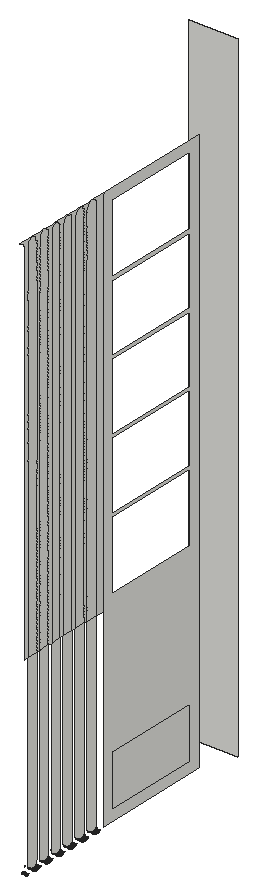
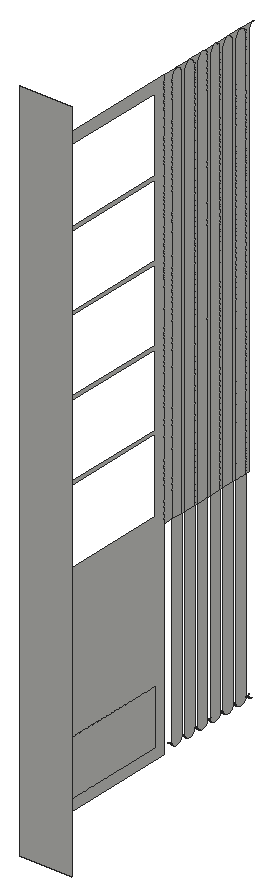
# SketchUp Ruby script. Lengths in inches.
U = 1.inch
M = Sketchup.active_model
def pt(a) = Geom::Point3d.new(a.map { |v| v * U })
def face(e, loops, mat)
  f = e.add_face(loops[0].map { |a| pt(a) })
  loops[1..].each { |l| e.add_face(l.map { |a| pt(a) }).erase! }
  f.material = f.back_material = mat if mat
  f
end
# faces: each face lists its corners as indices into pts; further lists are holes
def faces(e, pts, list, mat = nil) = list.each { |f| face(e, (f[0].is_a?(Array) ? f : [f]).map { |l| l.map { |i| pts[i] } }, mat) }
# xy, xz, yz: faces in a plane at the given z, y or x. An outline is a flat list of corners, or four numbers for a rectangle; further outlines are holes
def ring(l) = l.size == 4 ? [[l[0], l[1]], [l[2], l[1]], [l[2], l[3]], [l[0], l[3]]] : l.each_slice(2).to_a
def flat(e, list, mat, &to3) = list.each { |f| face(e, (f[0].is_a?(Array) ? f : [f]).map { |l| ring(l).map { |u, v| to3.(u, v) } }, mat) }
def xy(e, z, list, mat = nil) = flat(e, list, mat) { |x, y| [x, y, z] }
def xz(e, y, list, mat = nil) = flat(e, list, mat) { |x, z| [x, y, z] }
def yz(e, x, list, mat = nil) = flat(e, list, mat) { |y, z| [x, y, z] }
def lines(e, pts, list) = list.each { |a, b| e.add_line(pt(pts[a]), pt(pts[b])) }
# prism: a flat outline (further loops are holes) pulled along v
def prism(e, loops, v, mat = nil)
  f = face(e, loops, mat); d = Geom::Vector3d.new(v.map { |x| x * U })
  f.pushpull(f.normal.samedirection?(d) ? d.length : -d.length)
end
def box(e, o, s, mat = nil) = prism(e, [[o, [o[0] + s[0], o[1], o[2]], [o[0] + s[0], o[1] + s[1], o[2]], [o[0], o[1] + s[1], o[2]]]], [0, 0, s[2]], mat)
def at(x, y, z, deg = 0) = Geom::Transformation.translation(pt([x, y, z])) * Geom::Transformation.rotation(ORIGIN, Z_AXIS, deg.degrees)
def axes(o, x, y, z) = Geom::Transformation.new([*x, 0, *y, 0, *z, 0, *pt(o).to_a, 1])
def part(name) = M.definitions.add(name)
# library, detail: a bought-in or finely detailed component or shape, given as its bounding box
def library(name, o, s) = part(name).tap { |d| box(d.entities, o, s) }
def detail(e, o, s) = box(e.add_group.entities, o, s)
def put(e, d, t, mat = nil) = e.add_instance(d, t).tap { |i| i.material = mat if mat }
def group(e, t, mat = nil) = e.add_group.tap { |g| g.transformation = t; g.material = mat if mat }.entities
root = M.entities
xz(root,120,[[0,0,9,120]])
yz(root,9,[[[88.732,2,111,108],[90.732,40,109,52.9],[90.732,93.1,109,106],[90.732,79.9,109,92.5],[90.732,53.5,109,66.1],[90.732,66.7,109,79.3],[90.732,4,109,13.575]],[72.022,2.396,72.079,2.398,72.136,2.403,72.193,2.41,72.249,2.421,72.305,2.435,72.36,2.452,72.413,2.473,72.466,2.495,72.517,2.521,72.567,2.55,72.615,2.581,72.661,2.615,72.706,2.651,72.748,2.69,72.788,2.731,72.826,2.774,72.861,2.82,72.894,2.867,72.924,2.915,72.952,2.966,72.976,3.018,72.998,3.071,73.017,3.125,73.033,3.18,73.045,3.236,73.055,3.292,73.0625,3.363,73.0625,38,70.981,38,70.981,3.363,70.988,3.292,70.998,3.236,71.011,3.18,71.027,3.125,71.045,3.071,71.067,3.018,71.092,2.966,71.119,2.915,71.15,2.867,71.182,2.82,71.218,2.774,71.255,2.731,71.296,2.69,71.338,2.651,71.382,2.615,71.428,2.581,71.477,2.55,71.526,2.521,71.577,2.495,71.63,2.473,71.684,2.452,71.739,2.435,71.794,2.421,71.85,2.41,71.907,2.403,71.964,2.398],[74.809,2.396,74.867,2.398,74.924,2.403,74.981,2.41,75.037,2.421,75.092,2.435,75.147,2.452,75.201,2.473,75.254,2.495,75.305,2.521,75.354,2.55,75.403,2.581,75.449,2.615,75.493,2.651,75.535,2.69,75.576,2.731,75.613,2.774,75.649,2.82,75.681,2.867,75.712,2.915,75.739,2.966,75.764,3.018,75.786,3.071,75.804,3.125,75.82,3.18,75.833,3.236,75.843,3.292,75.85,3.363,75.85,38,73.768,38,73.768,3.363,73.776,3.292,73.786,3.236,73.798,3.18,73.814,3.125,73.833,3.071,73.855,3.018,73.879,2.966,73.907,2.915,73.937,2.867,73.97,2.82,74.005,2.774,74.043,2.731,74.083,2.69,74.125,2.651,74.17,2.615,74.216,2.581,74.264,2.55,74.314,2.521,74.365,2.495,74.418,2.473,74.471,2.452,74.526,2.435,74.582,2.421,74.638,2.41,74.695,2.403,74.752,2.398],[77.597,2.396,77.654,2.398,77.711,2.403,77.768,2.41,77.824,2.421,77.88,2.435,77.935,2.452,77.988,2.473,78.041,2.495,78.092,2.521,78.142,2.55,78.19,2.581,78.236,2.615,78.281,2.651,78.323,2.69,78.363,2.731,78.401,2.774,78.436,2.82,78.469,2.867,78.499,2.915,78.527,2.966,78.551,3.018,78.573,3.071,78.592,3.125,78.608,3.18,78.62,3.236,78.63,3.292,78.637,3.363,78.637,38,76.556,38,76.556,3.363,76.563,3.292,76.573,3.236,76.586,3.18,76.602,3.125,76.62,3.071,76.642,3.018,76.667,2.966,76.694,2.915,76.725,2.867,76.757,2.82,76.793,2.774,76.83,2.731,76.871,2.69,76.913,2.651,76.957,2.615,77.003,2.581,77.052,2.55,77.101,2.521,77.152,2.495,77.205,2.473,77.259,2.452,77.314,2.435,77.369,2.421,77.425,2.41,77.482,2.403,77.539,2.398],[80.384,2.396,80.442,2.398,80.499,2.403,80.556,2.41,80.612,2.421,80.667,2.435,80.722,2.452,80.776,2.473,80.829,2.495,80.88,2.521,80.929,2.55,80.978,2.581,81.024,2.615,81.068,2.651,81.11,2.69,81.151,2.731,81.188,2.774,81.224,2.82,81.256,2.867,81.287,2.915,81.314,2.966,81.339,3.018,81.361,3.071,81.379,3.125,81.395,3.18,81.408,3.236,81.418,3.292,81.425,3.363,81.425,38,79.343,38,79.343,3.363,79.351,3.292,79.361,3.236,79.373,3.18,79.389,3.125,79.408,3.071,79.43,3.018,79.454,2.966,79.482,2.915,79.512,2.867,79.545,2.82,79.58,2.774,79.618,2.731,79.658,2.69,79.7,2.651,79.745,2.615,79.791,2.581,79.839,2.55,79.889,2.521,79.94,2.495,79.993,2.473,80.046,2.452,80.101,2.435,80.157,2.421,80.213,2.41,80.27,2.403,80.327,2.398],
  [83.172,2.396,83.229,2.398,83.286,2.403,83.343,2.41,83.399,2.421,83.455,2.435,83.51,2.452,83.563,2.473,83.616,2.495,83.667,2.521,83.717,2.55,83.765,2.581,83.811,2.615,83.856,2.651,83.898,2.69,83.938,2.731,83.976,2.774,84.011,2.82,84.044,2.867,84.074,2.915,84.102,2.966,84.126,3.018,84.148,3.071,84.167,3.125,84.183,3.18,84.195,3.236,84.205,3.292,84.212,3.363,84.212,38,82.131,38,82.131,3.363,82.138,3.292,82.148,3.236,82.161,3.18,82.177,3.125,82.195,3.071,82.217,3.018,82.242,2.966,82.269,2.915,82.3,2.867,82.332,2.82,82.368,2.774,82.405,2.731,82.446,2.69,82.488,2.651,82.532,2.615,82.578,2.581,82.627,2.55,82.676,2.521,82.727,2.495,82.78,2.473,82.834,2.452,82.889,2.435,82.944,2.421,83,2.41,83.057,2.403,83.114,2.398],[85.959,2.396,86.017,2.398,86.074,2.403,86.131,2.41,86.187,2.421,86.242,2.435,86.297,2.452,86.351,2.473,86.404,2.495,86.455,2.521,86.504,2.55,86.553,2.581,86.599,2.615,86.643,2.651,86.685,2.69,86.726,2.731,86.763,2.774,86.799,2.82,86.831,2.867,86.862,2.915,86.889,2.966,86.914,3.018,86.936,3.071,86.954,3.125,86.97,3.18,86.983,3.236,86.993,3.292,87,3.363,87,38,84.918,38,84.918,3.363,84.926,3.292,84.936,3.236,84.948,3.18,84.964,3.125,84.983,3.071,85.005,3.018,85.029,2.966,85.057,2.915,85.087,2.867,85.12,2.82,85.155,2.774,85.193,2.731,85.233,2.69,85.275,2.651,85.32,2.615,85.366,2.581,85.414,2.55,85.464,2.521,85.515,2.495,85.568,2.473,85.621,2.452,85.676,2.435,85.732,2.421,85.788,2.41,85.845,2.403,85.902,2.398],[70.275,3.363,70.278,3.407,70.278,3.464,70.275,3.521],[70.981,3.363,70.981,3.521,70.978,3.464,70.978,3.407],[73.0625,3.363,73.065,3.407,73.065,3.464,73.0625,3.521],
  [73.768,3.363,73.768,3.521,73.766,3.464,73.766,3.407],[75.85,3.363,75.853,3.407,75.853,3.464,75.85,3.521],[76.556,3.363,76.556,3.521,76.553,3.464,76.553,3.407],[78.637,3.363,78.64,3.407,78.64,3.464,78.637,3.521],[79.343,3.363,79.343,3.521,79.341,3.464,79.341,3.407],
  [81.425,3.363,81.428,3.407,81.428,3.464,81.425,3.521],[82.131,3.363,82.131,3.521,82.128,3.464,82.128,3.407],[84.212,3.363,84.215,3.407,84.215,3.464,84.212,3.521],[84.918,3.363,84.918,3.521,84.916,3.464,84.916,3.407],[84.918,3.363,84.918,3.521,84.916,3.464,84.916,3.407],
  [87,3.363,87.003,3.407,87.003,3.464,87,3.521],[87,3.363,87.003,3.407,87.003,3.464,87,3.521],[90.732,4,109,13.575],[70.275,38,70.981,38,70.981,106.961,70.982,107.015,70.987,107.069,70.994,107.123,71.004,107.177,71.016,107.23,71.032,107.282,71.05,107.334,71.071,107.384,71.094,107.433,71.12,107.481,71.149,107.528,71.18,107.572,71.213,107.616,71.248,107.657,71.286,107.697,71.325,107.734,71.367,107.769,71.41,107.803,71.455,107.834,71.501,107.862,71.549,107.888,71.598,107.911,71.649,107.932,71.7,107.95,71.752,107.966,71.805,107.979,71.859,107.989,71.913,107.996,71.967,108,69.289,108,69.343,107.996,69.397,107.989,69.451,107.979,69.504,107.966,69.556,107.95,69.607,107.932,69.658,107.911,69.707,107.888,69.755,107.862,69.801,107.834,69.846,107.803,69.889,107.769,69.931,107.734,69.97,107.697,70.008,107.657,70.043,107.616,70.076,107.572,70.107,107.528,70.136,107.481,70.162,107.433,70.185,107.384,70.206,107.334,70.224,107.282,70.24,107.23,70.252,107.177,70.262,107.123,70.269,107.069,70.274,107.015,70.275,106.961],[70.981,38,73.0625,38,73.0625,106.961,73.061,107.015,73.057,107.069,73.05,107.123,73.04,107.177,73.027,107.23,73.012,107.282,72.993,107.334,72.973,107.384,72.949,107.433,72.923,107.481,72.895,107.528,72.864,107.572,72.831,107.616,72.795,107.657,72.758,107.697,72.718,107.734,72.677,107.769,72.633,107.803,72.589,107.834,72.542,107.862,72.494,107.888,72.445,107.911,72.395,107.932,72.343,107.95,72.291,107.966,72.238,107.979,72.185,107.989,72.131,107.996,72.076,108,71.967,108,71.913,107.996,71.859,107.989,71.805,107.979,71.752,107.966,71.7,107.95,71.649,107.932,71.598,107.911,71.549,107.888,71.501,107.862,71.455,107.834,71.41,107.803,71.367,107.769,71.325,107.734,71.286,107.697,71.248,107.657,71.213,107.616,71.18,107.572,71.149,107.528,71.12,107.481,71.094,107.433,71.071,107.384,71.05,107.334,71.032,107.282,71.016,107.23,71.004,107.177,70.994,107.123,70.987,107.069,70.982,107.015,70.981,106.961],
  [73.0625,38,73.768,38,73.768,106.961,73.77,107.015,73.774,107.069,73.781,107.123,73.791,107.177,73.804,107.23,73.819,107.282,73.838,107.334,73.858,107.384,73.882,107.433,73.908,107.481,73.936,107.528,73.967,107.572,74,107.616,74.036,107.657,74.073,107.697,74.113,107.734,74.154,107.769,74.198,107.803,74.242,107.834,74.289,107.862,74.337,107.888,74.386,107.911,74.436,107.932,74.488,107.95,74.54,107.966,74.593,107.979,74.646,107.989,74.7,107.996,74.755,108,72.076,108,72.131,107.996,72.185,107.989,72.238,107.979,72.291,107.966,72.343,107.95,72.395,107.932,72.445,107.911,72.494,107.888,72.542,107.862,72.589,107.834,72.633,107.803,72.677,107.769,72.718,107.734,72.758,107.697,72.795,107.657,72.831,107.616,72.864,107.572,72.895,107.528,72.923,107.481,72.949,107.433,72.973,107.384,72.993,107.334,73.012,107.282,73.027,107.23,73.04,107.177,73.05,107.123,73.057,107.069,73.061,107.015,73.0625,106.961],[73.768,38,75.85,38,75.85,106.961,75.849,107.015,75.844,107.069,75.837,107.123,75.827,107.177,75.815,107.23,75.799,107.282,75.781,107.334,75.76,107.384,75.737,107.433,75.711,107.481,75.682,107.528,75.651,107.572,75.618,107.616,75.583,107.657,75.545,107.697,75.506,107.734,75.464,107.769,75.421,107.803,75.376,107.834,75.33,107.862,75.282,107.888,75.233,107.911,75.182,107.932,75.131,107.95,75.079,107.966,75.026,107.979,74.972,107.989,74.918,107.996,74.864,108,74.755,108,74.7,107.996,74.646,107.989,74.593,107.979,74.54,107.966,74.488,107.95,74.436,107.932,74.386,107.911,74.337,107.888,74.289,107.862,74.242,107.834,74.198,107.803,74.154,107.769,74.113,107.734,74.073,107.697,74.036,107.657,74,107.616,73.967,107.572,73.936,107.528,73.908,107.481,73.882,107.433,73.858,107.384,73.838,107.334,73.819,107.282,73.804,107.23,73.791,107.177,73.781,107.123,73.774,107.069,73.77,107.015,73.768,106.961],[75.85,38,76.556,38,76.556,106.961,76.557,107.015,76.562,107.069,76.569,107.123,76.579,107.177,76.591,107.23,76.607,107.282,76.625,107.334,76.646,107.384,76.669,107.433,76.695,107.481,76.724,107.528,76.755,107.572,76.788,107.616,76.823,107.657,76.861,107.697,76.9,107.734,76.942,107.769,76.985,107.803,77.03,107.834,77.076,107.862,77.124,107.888,77.173,107.911,77.224,107.932,77.275,107.95,77.327,107.966,77.38,107.979,77.434,107.989,77.488,107.996,77.542,108,74.864,108,74.918,107.996,74.972,107.989,75.026,107.979,75.079,107.966,75.131,107.95,75.182,107.932,75.233,107.911,75.282,107.888,75.33,107.862,75.376,107.834,75.421,107.803,75.464,107.769,75.506,107.734,75.545,107.697,75.583,107.657,75.618,107.616,75.651,107.572,75.682,107.528,75.711,107.481,75.737,107.433,75.76,107.384,75.781,107.334,75.799,107.282,75.815,107.23,75.827,107.177,75.837,107.123,75.844,107.069,75.849,107.015,75.85,106.961],[76.556,38,78.637,38,78.637,106.961,78.636,107.015,78.632,107.069,78.625,107.123,78.615,107.177,78.602,107.23,78.587,107.282,78.568,107.334,78.548,107.384,78.524,107.433,78.498,107.481,78.47,107.528,78.439,107.572,78.406,107.616,78.37,107.657,78.333,107.697,78.293,107.734,78.252,107.769,78.208,107.803,78.164,107.834,78.117,107.862,78.069,107.888,78.02,107.911,77.97,107.932,77.918,107.95,77.866,107.966,77.813,107.979,77.76,107.989,77.706,107.996,77.651,108,77.542,108,77.488,107.996,77.434,107.989,77.38,107.979,77.327,107.966,77.275,107.95,77.224,107.932,77.173,107.911,77.124,107.888,77.076,107.862,77.03,107.834,76.985,107.803,76.942,107.769,76.9,107.734,76.861,107.697,76.823,107.657,76.788,107.616,76.755,107.572,76.724,107.528,76.695,107.481,76.669,107.433,76.646,107.384,76.625,107.334,76.607,107.282,76.591,107.23,76.579,107.177,76.569,107.123,76.562,107.069,76.557,107.015,76.556,106.961],[78.637,38,79.343,38,79.343,106.961,79.345,107.015,79.349,107.069,79.356,107.123,79.366,107.177,79.379,107.23,79.394,107.282,79.413,107.334,79.433,107.384,79.457,107.433,79.483,107.481,79.511,107.528,79.542,107.572,79.575,107.616,79.611,107.657,79.648,107.697,79.688,107.734,79.729,107.769,79.773,107.803,79.817,107.834,79.864,107.862,79.912,107.888,79.961,107.911,80.011,107.932,80.0625,107.95,80.115,107.966,80.168,107.979,80.221,107.989,80.275,107.996,80.33,108,77.651,108,77.706,107.996,77.76,107.989,77.813,107.979,77.866,107.966,77.918,107.95,77.97,107.932,78.02,107.911,78.069,107.888,78.117,107.862,78.164,107.834,78.208,107.803,78.252,107.769,78.293,107.734,78.333,107.697,78.37,107.657,78.406,107.616,78.439,107.572,78.47,107.528,78.498,107.481,78.524,107.433,78.548,107.384,78.568,107.334,78.587,107.282,78.602,107.23,78.615,107.177,78.625,107.123,78.632,107.069,78.636,107.015,78.637,106.961],
  [79.343,38,81.425,38,81.425,106.961,81.424,107.015,81.419,107.069,81.412,107.123,81.402,107.177,81.39,107.23,81.374,107.282,81.356,107.334,81.335,107.384,81.312,107.433,81.286,107.481,81.257,107.528,81.226,107.572,81.193,107.616,81.158,107.657,81.12,107.697,81.081,107.734,81.039,107.769,80.996,107.803,80.951,107.834,80.905,107.862,80.857,107.888,80.808,107.911,80.757,107.932,80.706,107.95,80.654,107.966,80.601,107.979,80.547,107.989,80.493,107.996,80.439,108,80.33,108,80.275,107.996,80.221,107.989,80.168,107.979,80.115,107.966,80.0625,107.95,80.011,107.932,79.961,107.911,79.912,107.888,79.864,107.862,79.817,107.834,79.773,107.803,79.729,107.769,79.688,107.734,79.648,107.697,79.611,107.657,79.575,107.616,79.542,107.572,79.511,107.528,79.483,107.481,79.457,107.433,79.433,107.384,79.413,107.334,79.394,107.282,79.379,107.23,79.366,107.177,79.356,107.123,79.349,107.069,79.345,107.015,79.343,106.961],[81.425,38,82.131,38,82.131,106.961,82.132,107.015,82.137,107.069,82.144,107.123,82.154,107.177,82.166,107.23,82.182,107.282,82.2,107.334,82.221,107.384,82.244,107.433,82.27,107.481,82.299,107.528,82.33,107.572,82.363,107.616,82.398,107.657,82.436,107.697,82.475,107.734,82.517,107.769,82.56,107.803,82.605,107.834,82.651,107.862,82.699,107.888,82.748,107.911,82.799,107.932,82.85,107.95,82.902,107.966,82.955,107.979,83.009,107.989,83.063,107.996,83.117,108,80.439,108,80.493,107.996,80.547,107.989,80.601,107.979,80.654,107.966,80.706,107.95,80.757,107.932,80.808,107.911,80.857,107.888,80.905,107.862,80.951,107.834,80.996,107.803,81.039,107.769,81.081,107.734,81.12,107.697,81.158,107.657,81.193,107.616,81.226,107.572,81.257,107.528,81.286,107.481,81.312,107.433,81.335,107.384,81.356,107.334,81.374,107.282,81.39,107.23,81.402,107.177,81.412,107.123,81.419,107.069,81.424,107.015,81.425,106.961],[82.131,38,84.212,38,84.212,106.961,84.211,107.015,84.207,107.069,84.2,107.123,84.19,107.177,84.177,107.23,84.162,107.282,84.143,107.334,84.123,107.384,84.099,107.433,84.073,107.481,84.045,107.528,84.014,107.572,83.981,107.616,83.945,107.657,83.908,107.697,83.868,107.734,83.827,107.769,83.783,107.803,83.739,107.834,83.692,107.862,83.644,107.888,83.595,107.911,83.545,107.932,83.493,107.95,83.441,107.966,83.388,107.979,83.335,107.989,83.281,107.996,83.226,108,83.117,108,83.063,107.996,83.009,107.989,82.955,107.979,82.902,107.966,82.85,107.95,82.799,107.932,82.748,107.911,82.699,107.888,82.651,107.862,82.605,107.834,82.56,107.803,82.517,107.769,82.475,107.734,82.436,107.697,82.398,107.657,82.363,107.616,82.33,107.572,82.299,107.528,82.27,107.481,82.244,107.433,82.221,107.384,82.2,107.334,82.182,107.282,82.166,107.23,82.154,107.177,82.144,107.123,82.137,107.069,82.132,107.015,82.131,106.961],[84.212,38,84.918,38,84.918,106.961,84.92,107.015,84.924,107.069,84.931,107.123,84.941,107.177,84.954,107.23,84.969,107.282,84.988,107.334,85.008,107.384,85.032,107.433,85.058,107.481,85.086,107.528,85.117,107.572,85.15,107.616,85.186,107.657,85.223,107.697,85.263,107.734,85.304,107.769,85.348,107.803,85.392,107.834,85.439,107.862,85.487,107.888,85.536,107.911,85.586,107.932,85.638,107.95,85.69,107.966,85.743,107.979,85.796,107.989,85.85,107.996,85.905,108,83.226,108,83.281,107.996,83.335,107.989,83.388,107.979,83.441,107.966,83.493,107.95,83.545,107.932,83.595,107.911,83.644,107.888,83.692,107.862,83.739,107.834,83.783,107.803,83.827,107.769,83.868,107.734,83.908,107.697,83.945,107.657,83.981,107.616,84.014,107.572,84.045,107.528,84.073,107.481,84.099,107.433,84.123,107.384,84.143,107.334,84.162,107.282,84.177,107.23,84.19,107.177,84.2,107.123,84.207,107.069,84.211,107.015,84.212,106.961],[84.918,38,87,38,87,106.961,86.999,107.015,86.994,107.069,86.987,107.123,86.977,107.177,86.965,107.23,86.949,107.282,86.931,107.334,86.91,107.384,86.887,107.433,86.861,107.481,86.832,107.528,86.801,107.572,86.768,107.616,86.733,107.657,86.695,107.697,86.656,107.734,86.614,107.769,86.571,107.803,86.526,107.834,86.48,107.862,86.432,107.888,86.383,107.911,86.332,107.932,86.281,107.95,86.229,107.966,86.176,107.979,86.122,107.989,86.068,107.996,86.014,108,85.905,108,85.85,107.996,85.796,107.989,85.743,107.979,85.69,107.966,85.638,107.95,85.586,107.932,85.536,107.911,85.487,107.888,85.439,107.862,85.392,107.834,85.348,107.803,85.304,107.769,85.263,107.734,85.223,107.697,85.186,107.657,85.15,107.616,85.117,107.572,85.086,107.528,85.058,107.481,85.032,107.433,85.008,107.384,84.988,107.334,84.969,107.282,84.954,107.23,84.941,107.177,84.931,107.123,84.924,107.069,84.92,107.015,84.918,106.961],
  [87,38,88.732,38,88.732,108,86.014,108,86.068,107.996,86.122,107.989,86.176,107.979,86.229,107.966,86.281,107.95,86.332,107.932,86.383,107.911,86.432,107.888,86.48,107.862,86.526,107.834,86.571,107.803,86.614,107.769,86.656,107.734,86.695,107.697,86.733,107.657,86.768,107.616,86.801,107.572,86.832,107.528,86.861,107.481,86.887,107.433,86.91,107.384,86.931,107.334,86.949,107.282,86.965,107.23,86.977,107.177,86.987,107.123,86.994,107.069,86.999,107.015,87,106.961]])
p = [[9,71.684,2.452],[9,71.739,2.435],[10,71.739,2.435],[10,71.684,2.452],[9,71.794,2.421],[10,71.794,2.421],
  [9,71.85,2.41],[10,71.85,2.41],[9,71.907,2.403],[10,71.907,2.403],[9,71.964,2.398],[10,71.964,2.398],
  [9,72.022,2.396],[10,72.022,2.396],[9,72.079,2.398],[10,72.079,2.398],[9,72.136,2.403],[10,72.136,2.403],
  [9,72.193,2.41],[10,72.193,2.41],[9,72.249,2.421],[10,72.249,2.421],[9,72.305,2.435],[10,72.305,2.435],
  [9,72.36,2.452],[10,72.36,2.452],[9,74.471,2.452],[9,74.526,2.435],[10,74.526,2.435],[10,74.471,2.452],
  [9,74.582,2.421],[10,74.582,2.421],[9,74.638,2.41],[10,74.638,2.41],[9,74.695,2.403],[10,74.695,2.403],
  [9,74.752,2.398],[10,74.752,2.398],[9,74.809,2.396],[10,74.809,2.396],[9,74.867,2.398],[10,74.867,2.398],
  [9,74.924,2.403],[10,74.924,2.403],[9,74.981,2.41],[10,74.981,2.41],[9,75.037,2.421],[10,75.037,2.421],
  [9,75.092,2.435],[10,75.092,2.435],[9,75.147,2.452],[10,75.147,2.452],[9,77.259,2.452],[9,77.314,2.435],
  [10,77.314,2.435],[10,77.259,2.452],[9,77.369,2.421],[10,77.369,2.421],[9,77.425,2.41],[10,77.425,2.41],
  [9,77.482,2.403],[10,77.482,2.403],[9,77.539,2.398],[10,77.539,2.398],[9,77.597,2.396],[10,77.597,2.396],
  [9,77.654,2.398],[10,77.654,2.398],[9,77.711,2.403],[10,77.711,2.403],[9,77.768,2.41],[10,77.768,2.41],
  [9,77.824,2.421],[10,77.824,2.421],[9,77.88,2.435],[10,77.88,2.435],[9,77.935,2.452],[10,77.935,2.452],
  [9,80.046,2.452],[9,80.101,2.435],[10,80.101,2.435],[10,80.046,2.452],[9,80.157,2.421],[10,80.157,2.421],
  [9,80.213,2.41],[10,80.213,2.41],[9,80.27,2.403],[10,80.27,2.403],[9,80.327,2.398],[10,80.327,2.398],
  [9,80.384,2.396],[10,80.384,2.396],[9,80.442,2.398],[10,80.442,2.398],[9,80.499,2.403],[10,80.499,2.403],
  [9,80.556,2.41],[10,80.556,2.41],[9,80.612,2.421],[10,80.612,2.421],[9,80.667,2.435],[10,80.667,2.435],
  [9,80.722,2.452],[10,80.722,2.452],[9,82.834,2.452],[9,82.889,2.435],[10,82.889,2.435],[10,82.834,2.452],
  [9,82.944,2.421],[10,82.944,2.421],[9,83,2.41],[10,83,2.41],[9,83.057,2.403],[10,83.057,2.403],
  [9,83.114,2.398],[10,83.114,2.398],[9,83.172,2.396],[10,83.172,2.396],[9,83.229,2.398],[10,83.229,2.398],
  [9,83.286,2.403],[10,83.286,2.403],[9,83.343,2.41],[10,83.343,2.41],[9,83.399,2.421],[10,83.399,2.421],
  [9,83.455,2.435],[10,83.455,2.435],[9,83.51,2.452],[10,83.51,2.452],[9,85.621,2.452],[9,85.676,2.435],
  [10,85.676,2.435],[10,85.621,2.452],[9,85.732,2.421],[10,85.732,2.421],[9,85.788,2.41],[10,85.788,2.41],
  [9,85.845,2.403],[10,85.845,2.403],[9,85.902,2.398],[10,85.902,2.398],[9,85.959,2.396],[10,85.959,2.396],
  [9,86.017,2.398],[10,86.017,2.398],[9,86.074,2.403],[10,86.074,2.403],[9,86.131,2.41],[10,86.131,2.41],
  [9,86.187,2.421],[10,86.187,2.421],[9,86.242,2.435],[10,86.242,2.435],[9,86.297,2.452],[10,86.297,2.452],
  [9,69.572,2.452],[9,69.626,2.473],[10,69.626,2.473],[10,69.572,2.452],[9,69.679,2.495],[10,69.679,2.495],
  [9,69.73,2.521],[10,69.73,2.521],[9,69.779,2.55],[10,69.779,2.55],[9,69.828,2.581],[10,69.828,2.581],
  [9,71.428,2.581],[9,71.477,2.55],[10,71.477,2.55],[10,71.428,2.581],[9,71.526,2.521],[10,71.526,2.521],
  [9,71.577,2.495],[10,71.577,2.495],[9,71.63,2.473],[10,71.63,2.473],[9,72.413,2.473],[10,72.413,2.473],
  [9,72.466,2.495],[10,72.466,2.495],[9,72.517,2.521],[10,72.517,2.521],[9,72.567,2.55],[10,72.567,2.55],
  [9,72.615,2.581],[10,72.615,2.581],[9,74.216,2.581],[9,74.264,2.55],[10,74.264,2.55],[10,74.216,2.581],
  [9,74.314,2.521],[10,74.314,2.521],[9,74.365,2.495],[10,74.365,2.495],[9,74.418,2.473],[10,74.418,2.473],
  [9,75.201,2.473],[10,75.201,2.473],[9,75.254,2.495],[10,75.254,2.495],[9,75.305,2.521],[10,75.305,2.521],
  [9,75.354,2.55],[10,75.354,2.55],[9,75.403,2.581],[10,75.403,2.581],[9,77.003,2.581],[9,77.052,2.55],
  [10,77.052,2.55],[10,77.003,2.581],[9,77.101,2.521],[10,77.101,2.521],[9,77.152,2.495],[10,77.152,2.495],
  [9,77.205,2.473],[10,77.205,2.473],[9,77.988,2.473],[10,77.988,2.473],[9,78.041,2.495],[10,78.041,2.495],
  [9,78.092,2.521],[10,78.092,2.521],[9,78.142,2.55],[10,78.142,2.55],[9,78.19,2.581],[10,78.19,2.581],
  [9,79.791,2.581],[9,79.839,2.55],[10,79.839,2.55],[10,79.791,2.581],[9,79.889,2.521],[10,79.889,2.521],
  [9,79.94,2.495],[10,79.94,2.495],[9,79.993,2.473],[10,79.993,2.473],[9,80.776,2.473],[10,80.776,2.473],
  [9,80.829,2.495],[10,80.829,2.495],[9,80.88,2.521],[10,80.88,2.521],[9,80.929,2.55],[10,80.929,2.55],
  [9,80.978,2.581],[10,80.978,2.581],[9,82.578,2.581],[9,82.627,2.55],[10,82.627,2.55],[10,82.578,2.581],
  [9,82.676,2.521],[10,82.676,2.521],[9,82.727,2.495],[10,82.727,2.495],[9,82.78,2.473],[10,82.78,2.473],
  [9,83.563,2.473],[10,83.563,2.473],[9,83.616,2.495],[10,83.616,2.495],[9,83.667,2.521],[10,83.667,2.521],
  [9,83.717,2.55],[10,83.717,2.55],[9,83.765,2.581],[10,83.765,2.581],[9,85.366,2.581],[9,85.414,2.55],
  [10,85.414,2.55],[10,85.366,2.581],[9,85.464,2.521],[10,85.464,2.521],[9,85.515,2.495],[10,85.515,2.495],
  [9,85.568,2.473],[10,85.568,2.473],[9,86.351,2.473],[10,86.351,2.473],[9,86.404,2.495],[10,86.404,2.495],
  [9,86.455,2.521],[10,86.455,2.521],[9,86.504,2.55],[10,86.504,2.55],[9,86.553,2.581],[10,86.553,2.581],
  [9,69.874,2.615],[10,69.874,2.615],[9,69.918,2.651],[10,69.918,2.651],[9,71.338,2.651],[9,71.382,2.615],
  [10,71.382,2.615],[10,71.338,2.651],[9,72.661,2.615],[10,72.661,2.615],[9,72.706,2.651],[10,72.706,2.651],
  [9,74.125,2.651],[9,74.17,2.615],[10,74.17,2.615],[10,74.125,2.651],[9,75.449,2.615],[10,75.449,2.615],
  [9,75.493,2.651],[10,75.493,2.651],[9,76.913,2.651],[9,76.957,2.615],[10,76.957,2.615],[10,76.913,2.651],
  [9,78.236,2.615],[10,78.236,2.615],[9,78.281,2.651],[10,78.281,2.651],[9,79.7,2.651],[9,79.745,2.615],
  [10,79.745,2.615],[10,79.7,2.651],[9,81.024,2.615],[10,81.024,2.615],[9,81.068,2.651],[10,81.068,2.651],
  [9,82.488,2.651],[9,82.532,2.615],[10,82.532,2.615],[10,82.488,2.651],[9,83.811,2.615],[10,83.811,2.615],
  [9,83.856,2.651],[10,83.856,2.651],[9,85.275,2.651],[9,85.32,2.615],[10,85.32,2.615],[10,85.275,2.651],
  [9,86.599,2.615],[10,86.599,2.615],[9,86.643,2.651],[10,86.643,2.651],[9,69.96,2.69],[10,69.96,2.69],
  [9,70.001,2.731],[10,70.001,2.731],[9,71.255,2.731],[9,71.296,2.69],[10,71.296,2.69],[10,71.255,2.731],
  [9,72.748,2.69],[10,72.748,2.69],[9,72.788,2.731],[10,72.788,2.731],[9,74.043,2.731],[9,74.083,2.69],
  [10,74.083,2.69],[10,74.043,2.731],[9,75.535,2.69],[10,75.535,2.69],[9,75.576,2.731],[10,75.576,2.731],
  [9,76.83,2.731],[9,76.871,2.69],[10,76.871,2.69],[10,76.83,2.731],[9,78.323,2.69],[10,78.323,2.69],
  [9,78.363,2.731],[10,78.363,2.731],[9,79.618,2.731],[9,79.658,2.69],[10,79.658,2.69],[10,79.618,2.731],
  [9,81.11,2.69],[10,81.11,2.69],[9,81.151,2.731],[10,81.151,2.731],[9,82.405,2.731],[9,82.446,2.69],
  [10,82.446,2.69],[10,82.405,2.731],[9,83.898,2.69],[10,83.898,2.69],[9,83.938,2.731],[10,83.938,2.731],
  [9,85.193,2.731],[9,85.233,2.69],[10,85.233,2.69],[10,85.193,2.731],[9,86.685,2.69],[10,86.685,2.69],
  [9,86.726,2.731],[10,86.726,2.731]]
faces(root,p,[[0,1,2,3],[1,4,5,2],[4,6,7,5],[6,8,9,7],[8,10,11,9],[10,12,13,11],[12,14,15,13],[14,16,17,15],
  [16,18,19,17],[18,20,21,19],[20,22,23,21],[22,24,25,23],[26,27,28,29],[27,30,31,28],[30,32,33,31],[32,34,35,33],
  [34,36,37,35],[36,38,39,37],[38,40,41,39],[40,42,43,41],[42,44,45,43],[44,46,47,45],[46,48,49,47],[48,50,51,49],
  [52,53,54,55],[53,56,57,54],[56,58,59,57],[58,60,61,59],[60,62,63,61],[62,64,65,63],[64,66,67,65],[66,68,69,67],
  [68,70,71,69],[70,72,73,71],[72,74,75,73],[74,76,77,75],[78,79,80,81],[79,82,83,80],[82,84,85,83],[84,86,87,85],
  [86,88,89,87],[88,90,91,89],[90,92,93,91],[92,94,95,93],[94,96,97,95],[96,98,99,97],[98,100,101,99],[100,102,103,101],
  [104,105,106,107],[105,108,109,106],[108,110,111,109],[110,112,113,111],[112,114,115,113],[114,116,117,115],[116,118,119,117],[118,120,121,119],
  [120,122,123,121],[122,124,125,123],[124,126,127,125],[126,128,129,127],[130,131,132,133],[131,134,135,132],[134,136,137,135],[136,138,139,137],
  [138,140,141,139],[140,142,143,141],[142,144,145,143],[144,146,147,145],[146,148,149,147],[148,150,151,149],[150,152,153,151],[152,154,155,153],
  [156,157,158,159],[157,160,161,158],[160,162,163,161],[162,164,165,163],[164,166,167,165],[168,169,170,171],[169,172,173,170],[172,174,175,173],
  [174,176,177,175],[176,0,3,177],[24,178,179,25],[178,180,181,179],[180,182,183,181],[182,184,185,183],[184,186,187,185],[188,189,190,191],
  [189,192,193,190],[192,194,195,193],[194,196,197,195],[196,26,29,197],[50,198,199,51],[198,200,201,199],[200,202,203,201],[202,204,205,203],
  [204,206,207,205],[208,209,210,211],[209,212,213,210],[212,214,215,213],[214,216,217,215],[216,52,55,217],[76,218,219,77],[218,220,221,219],
  [220,222,223,221],[222,224,225,223],[224,226,227,225],[228,229,230,231],[229,232,233,230],[232,234,235,233],[234,236,237,235],[236,78,81,237],
  [102,238,239,103],[238,240,241,239],[240,242,243,241],[242,244,245,243],[244,246,247,245],[248,249,250,251],[249,252,253,250],[252,254,255,253],
  [254,256,257,255],[256,104,107,257],[128,258,259,129],[258,260,261,259],[260,262,263,261],[262,264,265,263],[264,266,267,265],[268,269,270,271],
  [269,272,273,270],[272,274,275,273],[274,276,277,275],[276,130,133,277],[154,278,279,155],[278,280,281,279],[280,282,283,281],[282,284,285,283],
  [284,286,287,285],[166,288,289,167],[288,290,291,289],[292,293,294,295],[293,168,171,294],[186,296,297,187],[296,298,299,297],[300,301,302,303],
  [301,188,191,302],[206,304,305,207],[304,306,307,305],[308,309,310,311],[309,208,211,310],[226,312,313,227],[312,314,315,313],[316,317,318,319],
  [317,228,231,318],[246,320,321,247],[320,322,323,321],[324,325,326,327],[325,248,251,326],[266,328,329,267],[328,330,331,329],[332,333,334,335],
  [333,268,271,334],[286,336,337,287],[336,338,339,337],[290,340,341,291],[340,342,343,341],[344,345,346,347],[345,292,295,346],[298,348,349,299],
  [348,350,351,349],[352,353,354,355],[353,300,303,354],[306,356,357,307],[356,358,359,357],[360,361,362,363],[361,308,311,362],[314,364,365,315],
  [364,366,367,365],[368,369,370,371],[369,316,319,370],[322,372,373,323],[372,374,375,373],[376,377,378,379],[377,324,327,378],[330,380,381,331],
  [380,382,383,381],[384,385,386,387],[385,332,335,386],[338,388,389,339],[388,390,391,389]])
